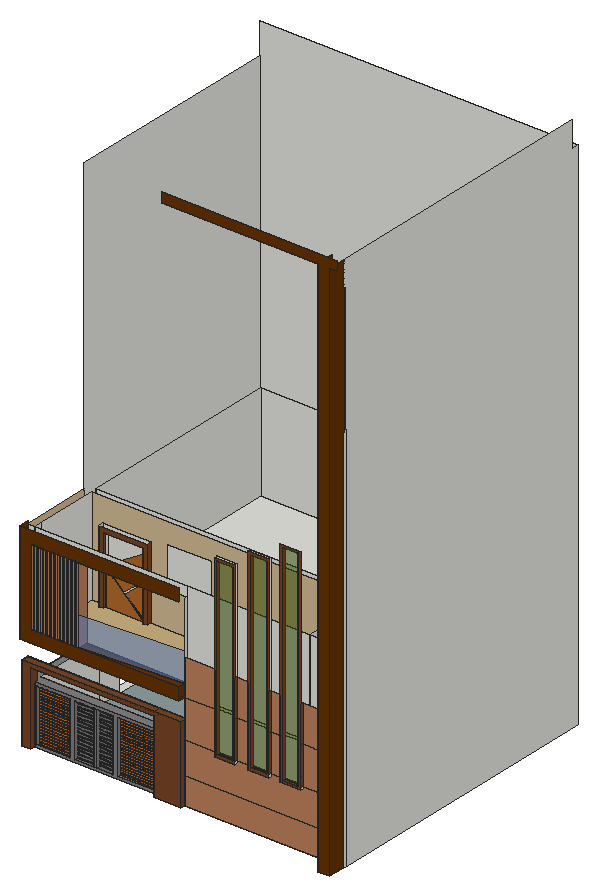
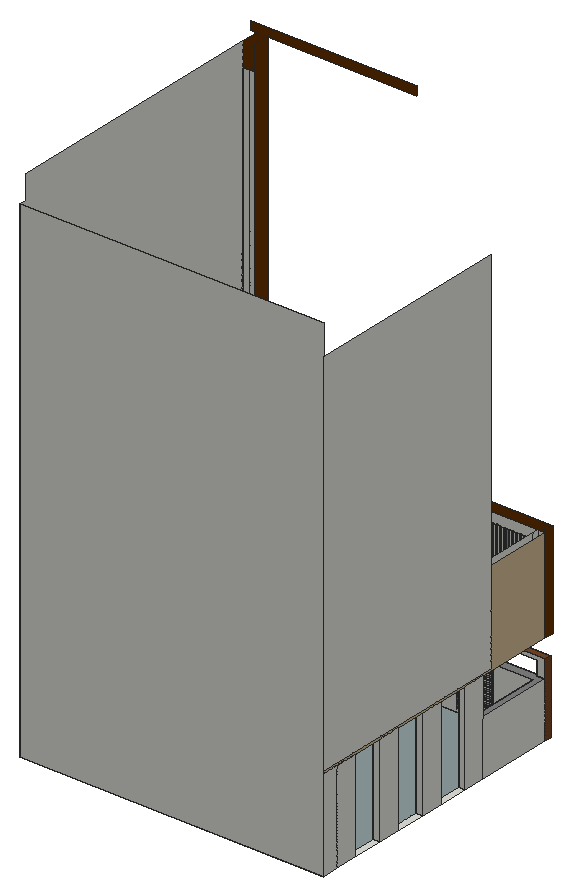
# SketchUp Ruby script. Lengths in inches.
U = 1.inch
M = Sketchup.active_model
def pt(a) = Geom::Point3d.new(a.map { |v| v * U })
def face(e, loops, mat)
  f = e.add_face(loops[0].map { |a| pt(a) })
  loops[1..].each { |l| e.add_face(l.map { |a| pt(a) }).erase! }
  f.material = f.back_material = mat if mat
  f
end
# faces: each face lists its corners as indices into pts; further lists are holes
def faces(e, pts, list, mat = nil) = list.each { |f| face(e, (f[0].is_a?(Array) ? f : [f]).map { |l| l.map { |i| pts[i] } }, mat) }
# xy, xz, yz: faces in a plane at the given z, y or x. An outline is a flat list of corners, or four numbers for a rectangle; further outlines are holes
def ring(l) = l.size == 4 ? [[l[0], l[1]], [l[2], l[1]], [l[2], l[3]], [l[0], l[3]]] : l.each_slice(2).to_a
def flat(e, list, mat, &to3) = list.each { |f| face(e, (f[0].is_a?(Array) ? f : [f]).map { |l| ring(l).map { |u, v| to3.(u, v) } }, mat) }
def xy(e, z, list, mat = nil) = flat(e, list, mat) { |x, y| [x, y, z] }
def xz(e, y, list, mat = nil) = flat(e, list, mat) { |x, z| [x, y, z] }
def yz(e, x, list, mat = nil) = flat(e, list, mat) { |y, z| [x, y, z] }
def lines(e, pts, list) = list.each { |a, b| e.add_line(pt(pts[a]), pt(pts[b])) }
# prism: a flat outline (further loops are holes) pulled along v
def prism(e, loops, v, mat = nil)
  f = face(e, loops, mat); d = Geom::Vector3d.new(v.map { |x| x * U })
  f.pushpull(f.normal.samedirection?(d) ? d.length : -d.length)
end
def box(e, o, s, mat = nil) = prism(e, [[o, [o[0] + s[0], o[1], o[2]], [o[0] + s[0], o[1] + s[1], o[2]], [o[0], o[1] + s[1], o[2]]]], [0, 0, s[2]], mat)
def at(x, y, z, deg = 0) = Geom::Transformation.translation(pt([x, y, z])) * Geom::Transformation.rotation(ORIGIN, Z_AXIS, deg.degrees)
def axes(o, x, y, z) = Geom::Transformation.new([*x, 0, *y, 0, *z, 0, *pt(o).to_a, 1])
def part(name) = M.definitions.add(name)
# library, detail: a bought-in or finely detailed component or shape, given as its bounding box
def library(name, o, s) = part(name).tap { |d| box(d.entities, o, s) }
def detail(e, o, s) = box(e.add_group.entities, o, s)
def put(e, d, t, mat = nil) = e.add_instance(d, t).tap { |i| i.material = mat if mat }
def group(e, t, mat = nil) = e.add_group.tap { |g| g.transformation = t; g.material = mat if mat }.entities
root = M.entities
M.materials.add("[0041_Chocolate]").color = [210, 105, 30]
M.materials.add("[0133_Gray]").color = [128, 128, 128]
M.materials.add("[0134_DimGray]").color = [105, 105, 105]
M.materials.add("[Color C08]").color = [102, 51, 0]
M.materials.add("[Formica Beige]").color = [211, 187, 149]
M.materials.add("[Metal Panel]").color = [143, 157, 158]
M.materials.add("[Roofing Slate Tan]").color = [200, 175, 128]
M.materials.add("[Translucent Glass Blue]").color = [100, 149, 237]
M.materials["[Translucent Glass Blue]"].alpha = 0.5
M.materials.add("[Translucent Glass Dark Green]").color = [62, 91, 5]
M.materials["[Translucent Glass Dark Green]"].alpha = 0.5
M.materials.add("[Wood Bamboo]").color = [177, 105, 43]
M.materials.add("[Wood Veneer 01]").color = [120, 70, 37]
M.materials.add("[Wood Veneer 02]").color = [190, 128, 91]
xy(root,0,[[390.57,0,397.32,21.4375],[397.32,0,405.5,21.4375],[10.125,15.4375,21.13,24.4375],[174.23,15.4375,207.71,24.4375],[207.71,21.4375,405.5,24.4375],
  [361.125,24.4375,361.125,375.4375,190.3125,375.4375,190.3125,125.375,184.3125,125.375,184.3125,375.4375,19.125,375.4375,19.125,362.75,10.125,362.75,10.125,384.4375,405.5,384.4375,405.5,24.4375],[10.125,125.375,19.125,154.25],[190.3125,125.375,361.125,131.375],[190.3125,131.375,361.125,375.4375],[10.125,154.25,19.125,194.875],
  [10.125,194.875,19.125,223.75],[10.125,223.75,19.125,264.375],[10.125,264.375,19.125,293.25],[10.125,293.25,19.125,333.875],[10.125,333.875,19.125,362.75]])
xy(root,0,[[21.13,21.4375,21.13,24.4375,10.125,24.4375,10.125,125.375,19.125,125.375,19.125,33.4375,361.125,33.4375,361.125,24.4375,174.23,24.4375,174.23,21.4375]],"[0133_Gray]")
xy(root,0,[[19.125,33.4375,361.125,33.4375,361.125,125.375,184.3125,125.375,184.3125,375.4375,19.125,375.4375]],"[Metal Panel]")
xy(root,3,[[24.13,21.4375,65.12,24.4375],[124.17,21.4375,171.23,24.4375]],"[0133_Gray]")
xy(root,3,[[71.12,21.4375,94.64,41.6875],[98.04,21.4375,118.17,33.4375]],"[0134_DimGray]")
xy(root,4.0625,[[71.12,24.4375,94.64,41.6875]])
xy(root,4.84,[[98.04,24.4375,118.17,33.4375]])
xy(root,5.1,[[71.12,24.4375,94.64,33.4375]],"[0134_DimGray]")
xy(root,5.98,[[98.04,24.4375,118.17,33.4375]],"[0134_DimGray]")
xy(root,8.125,[[71.12,24.4375,94.64,33.4375]],"[0134_DimGray]")
xy(root,9,[[98.04,24.4375,118.17,33.4375]],"[0134_DimGray]")
xy(root,9.17,[[71.12,24.4375,94.64,33.4375]],"[0134_DimGray]")
xy(root,9.98,[[98.04,24.4375,118.17,33.4375]],"[0134_DimGray]")
xy(root,12.1875,[[71.12,24.4375,94.64,33.4375]],"[0134_DimGray]")
xy(root,13,[[98.04,24.4375,118.17,33.4375]],"[0134_DimGray]")
xy(root,13.23,[[71.12,24.4375,94.64,33.4375]],"[0134_DimGray]")
xy(root,13.98,[[98.04,24.4375,118.17,33.4375]],"[0134_DimGray]")
xy(root,16.25,[[71.12,24.4375,94.64,33.4375]],"[0134_DimGray]")
xy(root,17,[[98.04,24.4375,118.17,33.4375]],"[0134_DimGray]")
xy(root,17.29,[[71.12,24.4375,94.64,33.4375]],"[0134_DimGray]")
xy(root,17.98,[[98.04,24.4375,118.17,33.4375]],"[0134_DimGray]")
xy(root,20.3125,[[71.12,24.4375,94.64,33.4375]],"[0134_DimGray]")
xy(root,21,[[98.04,24.4375,118.17,33.4375]],"[0134_DimGray]")
xy(root,21.35,[[71.12,24.4375,94.64,33.4375]],"[0134_DimGray]")
xy(root,21.98,[[98.04,24.4375,118.17,33.4375]],"[0134_DimGray]")
xy(root,24.375,[[71.12,24.4375,94.64,33.4375]],"[0134_DimGray]")
xy(root,25,[[98.04,24.4375,118.17,33.4375]],"[0134_DimGray]")
xy(root,25.42,[[71.12,24.4375,94.64,33.4375]],"[0134_DimGray]")
xy(root,25.98,[[98.04,24.4375,118.17,33.4375]],"[0134_DimGray]")
xy(root,28.4375,[[71.12,24.4375,94.64,33.4375]],"[0134_DimGray]")
xy(root,29,[[98.04,24.4375,118.17,33.4375]],"[0134_DimGray]")
xy(root,29.48,[[71.12,24.4375,94.64,33.4375]],"[0134_DimGray]")
xy(root,29.98,[[98.04,24.4375,118.17,33.4375]],"[0134_DimGray]")
xy(root,32.5,[[71.12,24.4375,94.64,33.4375]],"[0134_DimGray]")
xy(root,33,[[98.04,24.4375,118.17,33.4375]],"[0134_DimGray]")
xy(root,33.54,[[71.12,24.4375,94.64,33.4375]],"[0134_DimGray]")
xy(root,33.98,[[98.04,24.4375,118.17,33.4375]],"[0134_DimGray]")
xy(root,36.5625,[[71.12,24.4375,94.64,33.4375]],"[0134_DimGray]")
xy(root,37,[[98.04,24.4375,118.17,33.4375]],"[0134_DimGray]")
xy(root,37.6,[[71.12,24.4375,94.64,33.4375]],"[0134_DimGray]")
xy(root,37.98,[[98.04,24.4375,118.17,33.4375]],"[0134_DimGray]")
xy(root,40.625,[[71.12,24.4375,94.64,33.4375]],"[0134_DimGray]")
xy(root,41,[[98.04,24.4375,118.17,33.4375]],"[0134_DimGray]")
xy(root,41.67,[[71.12,24.4375,94.64,33.4375]],"[0134_DimGray]")
xy(root,41.98,[[98.04,24.4375,118.17,33.4375]],"[0134_DimGray]")
xy(root,44.6875,[[71.12,24.4375,94.64,33.4375]],"[0134_DimGray]")
xy(root,45,[[98.04,24.4375,118.17,33.4375]],"[0134_DimGray]")
xy(root,45.73,[[71.12,24.4375,94.64,33.4375]],"[0134_DimGray]")
xy(root,45.98,[[98.04,24.4375,118.17,33.4375]],"[0134_DimGray]")
xy(root,48.75,[[71.12,24.4375,94.64,33.4375]],"[0134_DimGray]")
xy(root,49,[[98.04,24.4375,118.17,33.4375]],"[0134_DimGray]")
xy(root,49.79,[[71.12,24.4375,94.64,33.4375]],"[0134_DimGray]")
xy(root,49.98,[[98.04,24.4375,118.17,33.4375]],"[0134_DimGray]")
xy(root,52.8125,[[71.12,24.4375,94.64,33.4375]],"[0134_DimGray]")
xy(root,53,[[98.04,24.4375,118.17,33.4375]],"[0134_DimGray]")
xy(root,53.85,[[71.12,24.4375,94.64,33.4375]],"[0134_DimGray]")
xy(root,53.98,[[98.04,24.4375,118.17,33.4375]],"[0134_DimGray]")
xy(root,56.875,[[71.12,24.4375,94.64,33.4375]],"[0134_DimGray]")
xy(root,57,[[98.04,24.4375,118.17,33.4375]],"[0134_DimGray]")
xy(root,57.92,[[71.12,24.4375,94.64,33.4375]],"[0134_DimGray]")
xy(root,57.98,[[98.04,24.4375,118.17,33.4375]],"[0134_DimGray]")
xy(root,60.9375,[[71.12,24.4375,94.64,33.4375]],"[0134_DimGray]")
xy(root,61,[[98.04,24.4375,118.17,33.4375]],"[0134_DimGray]")
xy(root,61.98,[[71.12,24.4375,94.64,33.4375],[98.04,24.4375,118.17,33.4375]],"[0134_DimGray]")
xy(root,65,[[71.12,24.4375,94.64,33.4375],[98.04,24.4375,118.17,33.4375]],"[0134_DimGray]")
xy(root,65.98,[[98.04,24.4375,118.17,33.4375]])
xy(root,65.98,[[71.12,24.4375,94.64,33.4375]],"[0134_DimGray]")
xy(root,69,[[94.64,21.4375,98.04,24.4375]])
xy(root,69,[[24.13,21.4375,65.12,24.4375],[71.12,21.4375,94.64,33.4375],[98.04,21.4375,118.17,33.4375],[124.17,21.4375,171.23,24.4375]],"[0133_Gray]")
xy(root,69.68,[[247.53,18.4375,272.24,21.4375],[288.73,18.4375,314.74,21.4375],[328.65,18.4375,354.15,21.4375]],"[Wood Veneer 01]")
xy(root,72,[[21.13,21.4375,174.23,21.4375,174.23,24.4375,361.125,24.4375,361.125,33.4375,19.125,33.4375,19.125,125.375,10.125,125.375,10.125,24.4375,21.13,24.4375]],"[0133_Gray]")
xy(root,72.68,[[250.53,18.4375,269.24,21.4375],[291.73,18.4375,311.74,21.4375],[331.65,18.4375,351.15,21.4375]],"[Wood Veneer 01]")
xy(root,90.59,[[21.13,15.4375,174.23,24.4375]],"[Wood Veneer 01]")
xy(root,95.4375,[[10.125,15.4375,174.23,24.4375],[174.23,15.4375,207.71,24.4375]],"[Wood Veneer 01]")
xy(root,120,[[10.125,125.375,19.125,154.25],[10.125,194.875,19.125,223.75],[10.125,264.375,19.125,293.25],[10.125,333.875,19.125,362.75]])
xy(root,120,[[10.125,12.4375,207.71,24.4375]],"[Color C08]")
xy(root,120,[[10.125,24.4375,10.125,125.375,19.125,125.375,19.125,154.25,10.125,154.25,10.125,194.875,19.125,194.875,19.125,223.75,10.125,223.75,10.125,264.375,19.125,264.375,19.125,293.25,10.125,293.25,10.125,333.875,19.125,333.875,19.125,375.4375,184.3125,375.4375,184.3125,125.375,361.125,125.375,361.125,24.4375]],"[Formica Beige]")
xy(root,123,[[19.125,24.4375,361.125,33.4375],[33.28,106.4375,39.28,112.4375],[87.28,106.4375,93.28,112.4375],[39.28,109.4375,87.28,112.4375],[19.125,118.4375,361.125,375.4375]])
xy(root,123,[[19.125,33.4375,361.125,33.4375,361.125,112.4375,93.28,112.4375,93.28,106.4375,87.28,106.4375,87.28,109.4375,39.28,109.4375,39.28,106.4375,33.28,106.4375,33.28,112.4375,19.125,112.4375]],"[Roofing Slate Tan]")
xy(root,135.6875,[[25.48,12.4375,27.42,24.4375],[27.42,12.4375,31.24,24.4375],[31.24,12.4375,32.73,24.4375],[32.73,12.4375,36.55,24.4375],[36.55,12.4375,38.05,24.4375],
  [38.05,12.4375,41.86,24.4375],[41.86,12.4375,43.36,24.4375],[43.36,12.4375,47.17,24.4375],[47.17,12.4375,48.67,24.4375],[48.67,12.4375,52.49,24.4375],
  [52.49,12.4375,53.98,24.4375],[53.98,12.4375,57.8,24.4375],[57.8,12.4375,59.3,24.4375],[59.3,12.4375,63.11,24.4375],[63.11,12.4375,64.36,24.4375],
  [64.36,12.4375,68.17,24.4375],[68.17,12.4375,69.42,24.4375],[69.42,12.4375,73.24,24.4375],[73.24,12.4375,74.48,24.4375],[74.48,12.4375,78.3,24.4375],
  [78.3,12.4375,79.55,24.4375],[79.55,12.4375,83.36,24.4375]])
xy(root,135.6875,[[83.36,12.4375,207.71,12.4375,207.71,21.4375],[83.36,12.4375,207.71,21.4375,207.71,24.4375,83.36,24.4375]],"[Color C08]")
xz(root,0,[[390.57,0,405.5,0,405.5,676.625,413.3125,676.625,413.3125,688,196.46,688,196.46,676.625,390.57,676.625]],"[Color C08]")
xz(root,12.4375,[[10.125,120,207.71,120,207.71,135.6875,25.48,135.6875,25.48,230.45,207.71,230.45,207.71,246,10.125,246]],"[Color C08]")
xz(root,12.4375,[[27.42,135.6875,31.24,230.45],[32.73,135.6875,36.55,230.45],[38.05,135.6875,41.86,230.45],[43.36,135.6875,47.17,230.125],[48.67,135.6875,52.49,230.45],
  [53.98,135.6875,57.8,230.45],[59.3,135.6875,63.11,230.45],[64.36,135.6875,68.17,230.45],[69.42,135.6875,73.24,230.45],[74.48,135.6875,78.3,230.45],
  [79.55,135.6875,83.36,230.45]],"[Wood Veneer 02]")
xz(root,15.4375,[[10.125,0,21.13,0,21.13,90.59,174.23,90.59,174.23,0,207.71,0,207.71,95.4375,10.125,95.4375]],"[Wood Veneer 01]")
xz(root,18.4375,[[[247.53,69.68,272.24,291.38],[250.53,72.68,269.24,288.38]],[[288.73,69.68,314.74,312.99],[291.73,72.68,311.74,309.99]],[[328.65,69.68,354.15,335.47],[331.65,72.68,351.15,332.47]]],"[Wood Veneer 01]")
xz(root,21.4375,[[390.57,0,397.32,645],[397.32,0,405.5,645],[[247.53,69.68,272.24,291.38],[250.53,72.68,269.24,288.38]],[288.73,69.68,288.73,288.38,291.73,288.38,291.73,72.68,311.74,72.68,311.74,309.99,291.73,309.99,291.73,288.38,288.73,288.38,288.73,312.99,314.74,312.99,314.74,69.68]])
xz(root,21.4375,[[[21.13,0,174.23,72],[71.12,3,118.17,69],[124.17,3,171.23,69],[24.13,3,65.12,69]],[94.64,3,98.04,69]],"[0133_Gray]")
xz(root,21.4375,[[250.53,72.68,269.24,288.38],[291.73,72.68,311.74,309.99],[331.65,72.68,351.15,332.47]],"[Translucent Glass Dark Green]")
xz(root,21.4375,[[207.71,0,390.57,33.17],[207.71,33.17,390.57,33.17,390.57,72.68,354.15,72.68,354.15,69.68,328.65,69.68,328.65,72.68,314.74,72.68,314.74,69.68,288.73,69.68,288.73,72.68,272.24,72.68,272.24,69.68,247.53,69.68,247.53,72.68,207.71,72.68],[207.71,72.68,247.53,120],[272.24,72.68,288.73,120],[314.74,72.68,328.65,120],
  [354.15,72.68,390.57,120],[207.71,120,247.53,165.32],[272.24,120,288.73,165.32],[314.74,120,328.65,165.32],[354.15,120,390.57,165.32]],"[Wood Veneer 02]")
xz(root,24.4375,[[10.125,0,21.13,72],[174.23,0,207.71,72],[207.71,0,361.125,72],[361.125,0,405.5,123],[24.13,2.64,65.12,3],
  [124.17,3,171.23,3.03],[94.64,65.98,98.04,69],[10.125,72,10.125,95.4375,174.23,95.4375,174.23,90.59,21.13,90.59,21.13,72],[174.23,72,207.71,95.4375],[207.71,72,361.125,120],
  [10.125,120,10.125,243,19.125,243,19.125,123,207.71,123,207.71,120],[207.71,120,361.125,123],[19.125,123,19.125,243,207.71,243,207.71,230.45,25.48,230.45,25.48,123],[25.48,123,207.71,135.6875],[207.71,123,361.125,243],
  [361.125,123,405.5,243],[27.42,135.6875,31.24,230.45],[32.73,135.6875,36.55,230.45],[38.05,135.6875,41.86,230.45],[43.36,135.6875,47.17,230.125],
  [48.67,135.6875,52.49,230.45],[53.98,135.6875,57.8,230.45],[59.3,135.6875,63.11,230.45],[64.36,135.6875,68.17,230.45],[69.42,135.6875,73.24,230.45],
  [74.48,135.6875,78.3,230.45],[79.55,135.6875,83.36,230.45]])
xz(root,24.4375,[[24.13,3,65.12,4.875],[124.17,3.03,171.23,5.25],[24.13,4.875,65.12,6.01],[124.17,5.25,171.23,6.22],[24.13,6.01,65.12,8.25],
  [124.17,6.22,171.23,8.4375],[24.13,8.25,65.12,9.39],[124.17,8.4375,171.23,9.4],[24.13,9.39,65.12,11.625],[124.17,9.4,171.23,11.625],
  [24.13,11.625,65.12,12.76],[124.17,11.625,171.23,12.59],[124.17,12.59,171.23,14.8125],[24.13,12.76,65.12,15],[124.17,14.8125,171.23,15.78],
  [24.13,15,65.12,16.14],[124.17,15.78,171.23,18],[24.13,16.14,65.12,18.375],[124.17,18,171.23,18.97],[24.13,18.375,65.12,19.51],
  [124.17,18.97,171.23,21.1875],[24.13,19.51,65.12,21.75],[124.17,21.1875,171.23,22.15],[24.13,21.75,65.12,22.89],[124.17,22.15,171.23,24.375],
  [24.13,22.89,65.12,25.125],[124.17,24.375,171.23,25.34],[24.13,25.125,65.12,26.26],[124.17,25.34,171.23,27.5625],[24.13,26.26,65.12,28.5],
  [124.17,27.5625,171.23,28.53],[24.13,28.5,65.12,29.64],[124.17,28.53,171.23,30.75],[24.13,29.64,65.12,31.875],[124.17,30.75,171.23,31.72],
  [124.17,31.72,171.23,33.9375],[24.13,31.875,65.12,33.01],[24.13,33.01,65.12,35.25],[124.17,33.9375,171.23,34.9],[124.17,34.9,171.23,37.125],
  [24.13,35.25,65.12,36.39],[24.13,36.39,65.12,38.625],[124.17,37.125,171.23,38.09],[124.17,38.09,171.23,40.3125],[24.13,38.625,65.12,39.76],
  [24.13,39.76,65.12,42],[124.17,40.3125,171.23,41.28],[124.17,41.28,171.23,43.5],[24.13,42,65.12,43.14],[24.13,43.14,65.12,45.375],
  [124.17,43.5,171.23,44.47],[124.17,44.47,171.23,46.6875],[24.13,45.375,65.12,46.51],[24.13,46.51,65.12,48.75],[124.17,46.6875,171.23,47.65],
  [124.17,47.65,171.23,49.875],[24.13,48.75,65.12,49.89],[124.17,49.875,171.23,50.84],[24.13,49.89,65.12,52.125],[124.17,50.84,171.23,53.0625],
  [24.13,52.125,65.12,53.26],[124.17,53.0625,171.23,54.03],[24.13,53.26,65.12,55.5],[124.17,54.03,171.23,56.25],[24.13,55.5,65.12,56.64],
  [124.17,56.25,171.23,57.22],[24.13,56.64,65.12,58.875],[124.17,57.22,171.23,59.4375],[24.13,58.875,65.12,60.01],[124.17,59.4375,171.23,60.4],
  [24.13,60.01,65.12,62.25],[124.17,60.4,171.23,62.625],[24.13,62.25,65.12,63.39],[124.17,62.625,171.23,63.59],[24.13,63.39,65.12,65.625],
  [124.17,63.59,171.23,65.8125],[24.13,65.625,65.12,66.76],[124.17,65.8125,171.23,66.78],[24.13,66.76,65.12,69],[124.17,66.78,171.23,69]],"[0041_Chocolate]")
xz(root,24.4375,[[71.12,4.0625,94.64,5.1],[98.04,4.84,118.17,5.98],[71.12,8.125,94.64,9.17],[98.04,9,118.17,9.98],[71.12,12.1875,94.64,13.23],
  [98.04,13,118.17,13.98],[71.12,16.25,94.64,17.29],[98.04,17,118.17,17.98],[71.12,20.3125,94.64,21.35],[98.04,21,118.17,21.98],
  [71.12,24.375,94.64,25.42],[98.04,25,118.17,25.98],[71.12,28.4375,94.64,29.48],[98.04,29,118.17,29.98],[71.12,32.5,94.64,33.54],
  [98.04,33,118.17,33.98],[71.12,36.5625,94.64,37.6],[98.04,37,118.17,37.98],[71.12,40.625,94.64,41.67],[98.04,41,118.17,41.98],
  [71.12,44.6875,94.64,45.73],[98.04,45,118.17,45.98],[71.12,48.75,94.64,49.79],[98.04,49,118.17,49.98],[71.12,52.8125,94.64,53.85],
  [98.04,53,118.17,53.98],[71.12,56.875,94.64,57.92],[98.04,57,118.17,57.98],[71.12,60.9375,94.64,61.98],[98.04,61,118.17,61.98],
  [71.12,65,94.64,65.98],[98.04,65,118.17,65.98]],"[0134_DimGray]")
xz(root,33.4375,[[[19.125,0,361.125,72],[71.12,65.98,94.64,69],[71.12,61.98,94.64,65],[71.12,57.92,94.64,60.9375],[71.12,53.85,94.64,56.875],[71.12,49.79,94.64,52.8125],[71.12,45.73,94.64,48.75],[71.12,41.67,94.64,44.6875],[71.12,37.6,94.64,40.625],[71.12,33.54,94.64,36.5625],[71.12,29.48,94.64,32.5],[71.12,25.42,94.64,28.4375],[71.12,21.35,94.64,24.375],[71.12,17.29,94.64,20.3125],[71.12,13.23,94.64,16.25],[71.12,9.17,94.64,12.1875],[71.12,5.1,94.64,8.125],[98.04,5.98,118.17,9],[98.04,13.98,118.17,17],[98.04,65.98,118.17,69],[98.04,61.98,118.17,65],[98.04,57.98,118.17,61],[98.04,53.98,118.17,57],[98.04,49.98,118.17,53],[98.04,45.98,118.17,49],[98.04,41.98,118.17,45],[98.04,37.98,118.17,41],[98.04,33.98,118.17,37],[98.04,25.98,118.17,29],[98.04,21.98,118.17,25],[98.04,17.98,118.17,21],[98.04,9.98,118.17,13],[98.04,29.98,118.17,33],[98.04,3,118.17,4.84]]])
xz(root,41.6875,[[71.12,3,94.64,4.0625]])
xz(root,106.4375,[[33.28,123,39.28,123,39.28,207,87.28,207,87.28,123,93.28,123,93.28,213,33.28,213]],"[Wood Veneer 01]")
xz(root,109.4375,[[85.11,123,87.28,123,63.28,146.5,87.28,166.29,87.28,167.99,61.85,147.9,39.28,170,39.28,167.87]])
xz(root,109.4375,[[39.28,123,85.11,123,39.28,167.87],[87.28,123,87.28,166.29,63.28,146.5],[[61.85,147.9,87.28,167.99,87.28,198.61,39.28,170],[75.28,168.8,75.28,179.68,85.65,179.68,85.65,178.68,76.65,178.68,76.65,168.8]]],"[Wood Bamboo]")
xz(root,112.4375,[[33.28,123,33.28,213,93.28,213,93.28,123,87.28,123,87.28,207,39.28,207,39.28,123],[39.28,123,87.28,207]])
xz(root,112.4375,[[[19.125,123,33.28,123,33.28,213,93.28,213,93.28,123,361.125,123,361.125,243,19.125,243],[112.82,168.02,168.88,218.4]]],"[Formica Beige]")
xz(root,118.4375,[[19.125,123,361.125,243]])
xz(root,125.375,[[10.125,0,19.125,72],[184.3125,0,190.3125,120],[190.3125,0,361.125,120],[10.125,72,19.125,120]])
xz(root,154.25,[[10.125,0,19.125,120]])
xz(root,194.875,[[10.125,0,19.125,120]])
xz(root,223.75,[[10.125,0,19.125,120]])
xz(root,264.375,[[10.125,0,19.125,120]])
xz(root,293.25,[[10.125,0,19.125,120]])
xz(root,333.875,[[10.125,0,19.125,120]])
xz(root,362.75,[[10.125,0,19.125,120]])
xz(root,375.4375,[[19.125,0,184.3125,120],[190.3125,0,361.125,120],[19.125,123,361.125,243]])
xz(root,384.4375,[[10.125,0,405.5,645]])
yz(root,10.125,[[24.4375,0,125.375,72],[125.375,0,154.25,120],[194.875,0,223.75,120],[264.375,0,293.25,120],[333.875,0,362.75,120],
  [362.75,0,384.4375,120],[112.4375,123,384.4375,606]])
yz(root,10.125,[[12.4375,120,24.4375,246]],"[Color C08]")
yz(root,10.125,[[24.4375,120,24.4375,243,112.4375,243,112.4375,123,384.4375,123,384.4375,120]],"[Formica Beige]")
yz(root,10.125,[[15.4375,0,24.4375,95.4375]],"[Wood Veneer 01]")
yz(root,19.125,[[33.4375,0,125.375,72],[125.375,0,154.25,120],[194.875,0,223.75,120],[264.375,0,293.25,120],[333.875,0,362.75,120],
  [362.75,0,375.4375,120],[24.4375,123,33.4375,243],[33.4375,123,112.4375,243],[118.4375,123,375.4375,243]])
yz(root,21.13,[[21.4375,0,24.4375,72]])
yz(root,21.13,[[15.4375,0,21.4375,0,21.4375,72,24.4375,72,24.4375,90.59,15.4375,90.59]],"[Wood Veneer 01]")
yz(root,24.13,[[21.4375,3,24.4375,69]],"[0133_Gray]")
yz(root,25.48,[[12.4375,135.6875,24.4375,230.45]],"[Wood Veneer 02]")
yz(root,27.42,[[12.4375,135.6875,24.4375,230.45]],"[Wood Veneer 02]")
yz(root,31.24,[[12.4375,135.6875,24.4375,230.45]],"[Wood Veneer 02]")
yz(root,32.73,[[12.4375,135.6875,24.4375,230.45]],"[Wood Veneer 02]")
yz(root,33.28,[[106.4375,123,112.4375,213]])
yz(root,36.55,[[12.4375,135.6875,24.4375,230.45]],"[Wood Veneer 02]")
yz(root,38.05,[[12.4375,135.6875,24.4375,230.45]],"[Wood Veneer 02]")
yz(root,39.28,[[109.4375,123,112.4375,207]])
yz(root,39.28,[[106.4375,123,109.4375,207]],"[Wood Veneer 01]")
yz(root,41.86,[[12.4375,135.6875,24.4375,230.45]],"[Wood Veneer 02]")
yz(root,43.36,[[12.4375,135.6875,24.4375,230.125]],"[Wood Veneer 02]")
yz(root,47.17,[[12.4375,135.6875,24.4375,230.125]],"[Wood Veneer 02]")
yz(root,48.67,[[12.4375,135.6875,24.4375,230.45]],"[Wood Veneer 02]")
yz(root,52.49,[[12.4375,135.6875,24.4375,230.45]],"[Wood Veneer 02]")
yz(root,53.98,[[12.4375,135.6875,24.4375,230.45]],"[Wood Veneer 02]")
yz(root,57.8,[[12.4375,135.6875,24.4375,230.45]],"[Wood Veneer 02]")
yz(root,59.3,[[12.4375,135.6875,24.4375,230.45]],"[Wood Veneer 02]")
yz(root,63.11,[[12.4375,135.6875,24.4375,230.45]],"[Wood Veneer 02]")
yz(root,64.36,[[12.4375,135.6875,24.4375,230.45]],"[Wood Veneer 02]")
yz(root,65.12,[[21.4375,3,24.4375,69]],"[0133_Gray]")
yz(root,68.17,[[12.4375,135.6875,24.4375,230.45]],"[Wood Veneer 02]")
yz(root,69.42,[[12.4375,135.6875,24.4375,230.45]],"[Wood Veneer 02]")
yz(root,71.12,[[21.4375,3,41.6875,3,41.6875,4.0625,24.4375,4.0625,24.4375,5.1,33.4375,5.1,33.4375,8.125,24.4375,8.125,24.4375,9.17,33.4375,9.17,33.4375,12.1875,24.4375,12.1875,24.4375,13.23,33.4375,13.23,33.4375,16.25,24.4375,16.25,24.4375,17.29,33.4375,17.29,33.4375,20.3125,24.4375,20.3125,24.4375,21.35,33.4375,21.35,33.4375,24.375,24.4375,24.375,24.4375,25.42,33.4375,25.42,33.4375,28.4375,24.4375,28.4375,24.4375,29.48,33.4375,29.48,33.4375,32.5,24.4375,32.5,24.4375,33.54,33.4375,33.54,33.4375,36.5625,24.4375,36.5625,24.4375,37.6,33.4375,37.6,33.4375,40.625,24.4375,40.625,24.4375,41.67,33.4375,41.67,33.4375,44.6875,24.4375,44.6875,24.4375,45.73,33.4375,45.73,33.4375,48.75,24.4375,48.75,24.4375,49.79,33.4375,49.79,33.4375,52.8125,24.4375,52.8125,24.4375,53.85,33.4375,53.85,33.4375,56.875,24.4375,56.875,24.4375,57.92,33.4375,57.92,33.4375,60.9375,24.4375,60.9375,24.4375,61.98,33.4375,61.98,33.4375,65,24.4375,65,24.4375,65.98,33.4375,65.98,33.4375,69,21.4375,69]],"[0133_Gray]")
yz(root,73.24,[[12.4375,135.6875,24.4375,230.45]],"[Wood Veneer 02]")
yz(root,74.48,[[12.4375,135.6875,24.4375,230.45]],"[Wood Veneer 02]")
yz(root,78.3,[[12.4375,135.6875,24.4375,230.45]],"[Wood Veneer 02]")
yz(root,79.55,[[12.4375,135.6875,24.4375,230.45]],"[Wood Veneer 02]")
yz(root,83.36,[[12.4375,135.6875,24.4375,230.45]],"[Wood Veneer 02]")
yz(root,87.28,[[106.4375,123,109.4375,207],[109.4375,123,112.4375,207]])
yz(root,93.28,[[106.4375,123,112.4375,213]],"[Wood Veneer 01]")
yz(root,94.64,[[21.4375,3,21.4375,69,24.4375,69,24.4375,65,33.4375,65,33.4375,61.98,24.4375,61.98,24.4375,60.9375,33.4375,60.9375,33.4375,57.92,24.4375,57.92,24.4375,56.875,33.4375,56.875,33.4375,53.85,24.4375,53.85,24.4375,52.8125,33.4375,52.8125,33.4375,49.79,24.4375,49.79,24.4375,48.75,33.4375,48.75,33.4375,45.73,24.4375,45.73,24.4375,44.6875,33.4375,44.6875,33.4375,41.67,24.4375,41.67,24.4375,40.625,33.4375,40.625,33.4375,37.6,24.4375,37.6,24.4375,36.5625,33.4375,36.5625,33.4375,33.54,24.4375,33.54,24.4375,32.5,33.4375,32.5,33.4375,29.48,24.4375,29.48,24.4375,28.4375,33.4375,28.4375,33.4375,25.42,24.4375,25.42,24.4375,24.375,33.4375,24.375,33.4375,21.35,24.4375,21.35,24.4375,20.3125,33.4375,20.3125,33.4375,17.29,24.4375,17.29,24.4375,16.25,33.4375,16.25,33.4375,13.23,24.4375,13.23,24.4375,12.1875,33.4375,12.1875,33.4375,9.17,24.4375,9.17,24.4375,8.125,33.4375,8.125,33.4375,5.1,24.4375,5.1,24.4375,4.0625,41.6875,4.0625,41.6875,3],[24.4375,65.98,33.4375,69]],"[0133_Gray]")
yz(root,98.04,[[24.4375,65.98,33.4375,69]])
yz(root,98.04,[[21.4375,3,33.4375,3,33.4375,4.84,24.4375,4.84,24.4375,5.98,33.4375,5.98,33.4375,9,24.4375,9,24.4375,9.98,33.4375,9.98,33.4375,13,24.4375,13,24.4375,13.98,33.4375,13.98,33.4375,17,24.4375,17,24.4375,17.98,33.4375,17.98,33.4375,21,24.4375,21,24.4375,21.98,33.4375,21.98,33.4375,25,24.4375,25,24.4375,25.98,33.4375,25.98,33.4375,29,24.4375,29,24.4375,29.98,33.4375,29.98,33.4375,33,24.4375,33,24.4375,33.98,33.4375,33.98,33.4375,37,24.4375,37,24.4375,37.98,33.4375,37.98,33.4375,41,24.4375,41,24.4375,41.98,33.4375,41.98,33.4375,45,24.4375,45,24.4375,45.98,33.4375,45.98,33.4375,49,24.4375,49,24.4375,49.98,33.4375,49.98,33.4375,53,24.4375,53,24.4375,53.98,33.4375,53.98,33.4375,57,24.4375,57,24.4375,57.98,33.4375,57.98,33.4375,61,24.4375,61,24.4375,61.98,33.4375,61.98,33.4375,65,24.4375,65,24.4375,69,21.4375,69]],"[0133_Gray]")
yz(root,118.17,[[21.4375,3,21.4375,69,33.4375,69,33.4375,65.98,24.4375,65.98,24.4375,65,33.4375,65,33.4375,61.98,24.4375,61.98,24.4375,61,33.4375,61,33.4375,57.98,24.4375,57.98,24.4375,57,33.4375,57,33.4375,53.98,24.4375,53.98,24.4375,53,33.4375,53,33.4375,49.98,24.4375,49.98,24.4375,49,33.4375,49,33.4375,45.98,24.4375,45.98,24.4375,45,33.4375,45,33.4375,41.98,24.4375,41.98,24.4375,41,33.4375,41,33.4375,37.98,24.4375,37.98,24.4375,37,33.4375,37,33.4375,33.98,24.4375,33.98,24.4375,33,33.4375,33,33.4375,29.98,24.4375,29.98,24.4375,29,33.4375,29,33.4375,25.98,24.4375,25.98,24.4375,25,33.4375,25,33.4375,21.98,24.4375,21.98,24.4375,21,33.4375,21,33.4375,17.98,24.4375,17.98,24.4375,17,33.4375,17,33.4375,13.98,24.4375,13.98,24.4375,13,33.4375,13,33.4375,9.98,24.4375,9.98,24.4375,9,33.4375,9,33.4375,5.98,24.4375,5.98,24.4375,4.84,33.4375,4.84,33.4375,3]],"[0133_Gray]")
yz(root,124.17,[[21.4375,3,24.4375,69]],"[0133_Gray]")
yz(root,171.23,[[21.4375,3,24.4375,69]],"[0133_Gray]")
yz(root,174.23,[[21.4375,0,24.4375,72]])
yz(root,174.23,[[15.4375,0,15.4375,90.59,24.4375,90.59,24.4375,72,21.4375,72,21.4375,0]],"[Wood Veneer 01]")
yz(root,184.3125,[[125.375,0,375.4375,120]])
yz(root,190.3125,[[125.375,0,131.375,120],[131.375,0,375.4375,120]])
yz(root,207.71,[[21.4375,0,24.4375,72],[21.4375,72,24.4375,95.4375],[21.4375,95.4375,24.4375,120],[21.4375,120,24.4375,123],[21.4375,123,24.4375,135.6875],
  [21.4375,135.6875,24.4375,230.45]])
yz(root,207.71,[[12.4375,120,21.4375,123],[12.4375,123,21.4375,135.6875]],"[Color C08]")
yz(root,207.71,[[15.4375,0,21.4375,95.4375]],"[Wood Veneer 01]")
yz(root,247.53,[[18.4375,69.68,21.4375,72.68],[18.4375,72.68,21.4375,120],[18.4375,120,21.4375,165.32]],"[Wood Veneer 01]")
yz(root,250.53,[[18.4375,72.68,21.4375,288.38]],"[Wood Veneer 01]")
yz(root,269.24,[[18.4375,72.68,21.4375,288.38]],"[Wood Veneer 01]")
yz(root,272.24,[[18.4375,69.68,21.4375,72.68]])
yz(root,272.24,[[18.4375,72.68,21.4375,120],[18.4375,120,21.4375,165.32]],"[Wood Veneer 01]")
yz(root,288.73,[[18.4375,69.68,21.4375,72.68],[18.4375,72.68,21.4375,120],[18.4375,120,21.4375,165.32]],"[Wood Veneer 01]")
yz(root,291.73,[[18.4375,72.68,21.4375,309.99]],"[Wood Veneer 01]")
yz(root,311.74,[[18.4375,72.68,21.4375,309.99]],"[Wood Veneer 01]")
yz(root,314.74,[[18.4375,69.68,21.4375,72.68]])
yz(root,314.74,[[18.4375,72.68,21.4375,120],[18.4375,120,21.4375,165.32]],"[Wood Veneer 01]")
yz(root,328.65,[[18.4375,69.68,21.4375,72.68],[18.4375,72.68,21.4375,120],[18.4375,120,21.4375,165.32]],"[Wood Veneer 01]")
yz(root,331.65,[[18.4375,72.68,21.4375,332.47]],"[Wood Veneer 01]")
yz(root,351.15,[[18.4375,72.68,21.4375,332.47]],"[Wood Veneer 01]")
yz(root,354.15,[[18.4375,69.68,21.4375,72.68]])
yz(root,354.15,[[18.4375,72.68,21.4375,120],[18.4375,120,21.4375,165.32]],"[Wood Veneer 01]")
yz(root,361.125,[[24.4375,0,33.4375,72],[33.4375,0,125.375,120],[125.375,0,131.375,120],[131.375,0,375.4375,120],[24.4375,72,33.4375,120],
  [24.4375,123,112.4375,243],[118.4375,123,375.4375,243]])
yz(root,390.57,[[0,0,21.4375,676.625]],"[Color C08]")
yz(root,405.5,[[21.4375,0,24.4375,486],[24.4375,0,384.4375,0,384.4375,645,375.4375,645,375.4375,676.625,21.4375,676.625,21.4375,645,24.4375,645]])
yz(root,405.5,[[0,0,21.4375,676.625]],"[Color C08]")
p = [[83.36,12.4375,135.6875],[207.71,21.4375,135.6875],[207.71,21.4375,165.32],[207.71,21.4375,172.58],[83.36,12.4375,172.58],[361.125,33.4375,120],
  [370.125,33.4375,120],[361.125,131.375,120],[370.125,131.375,120],[19.125,375.4375,120],[19.125,375.4375,123],[25.48,12.4375,123],
  [25.48,24.4375,123],[85.11,109.4375,123],[87.28,109.4375,120.875],[24.13,24.4375,1.5],[65.12,24.4375,1.5],[124.17,24.4375,2.0625],
  [171.23,24.4375,2.0625],[94.64,24.4375,1.04],[71.12,24.4375,1.04],[94.64,24.4375,3],[71.12,24.4375,3]]
faces(root,p,[[0,1,2,3,4]],"[Translucent Glass Blue]")
lines(root,p,[[5,6],[7,8],[9,10],[11,12],[13,14],[15,16],[17,18],[19,20],[19,21],[22,20]])
